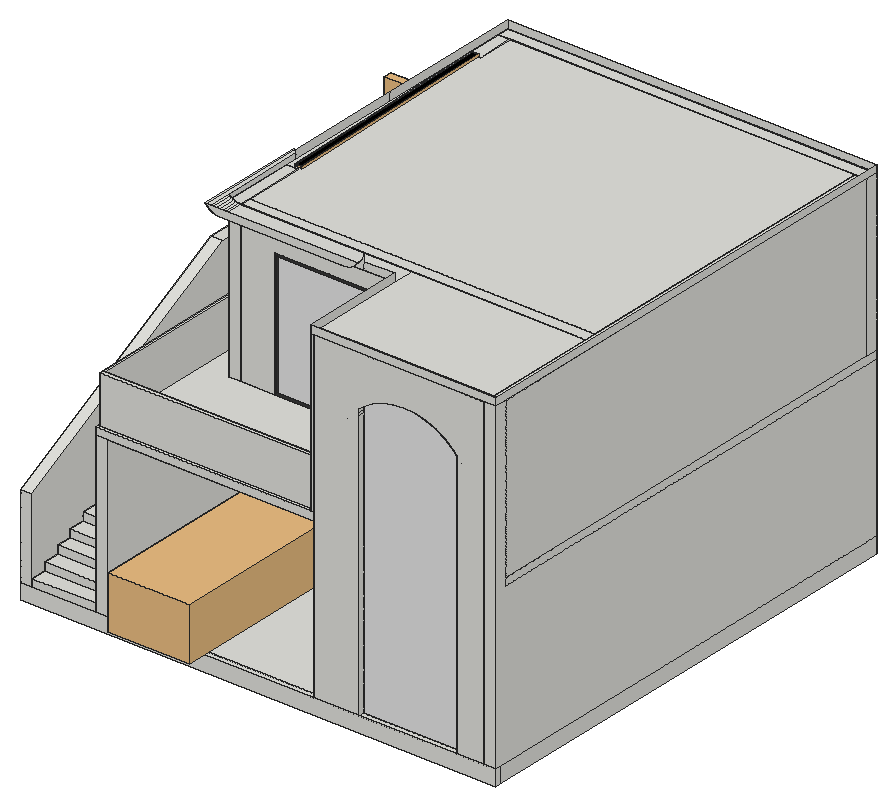
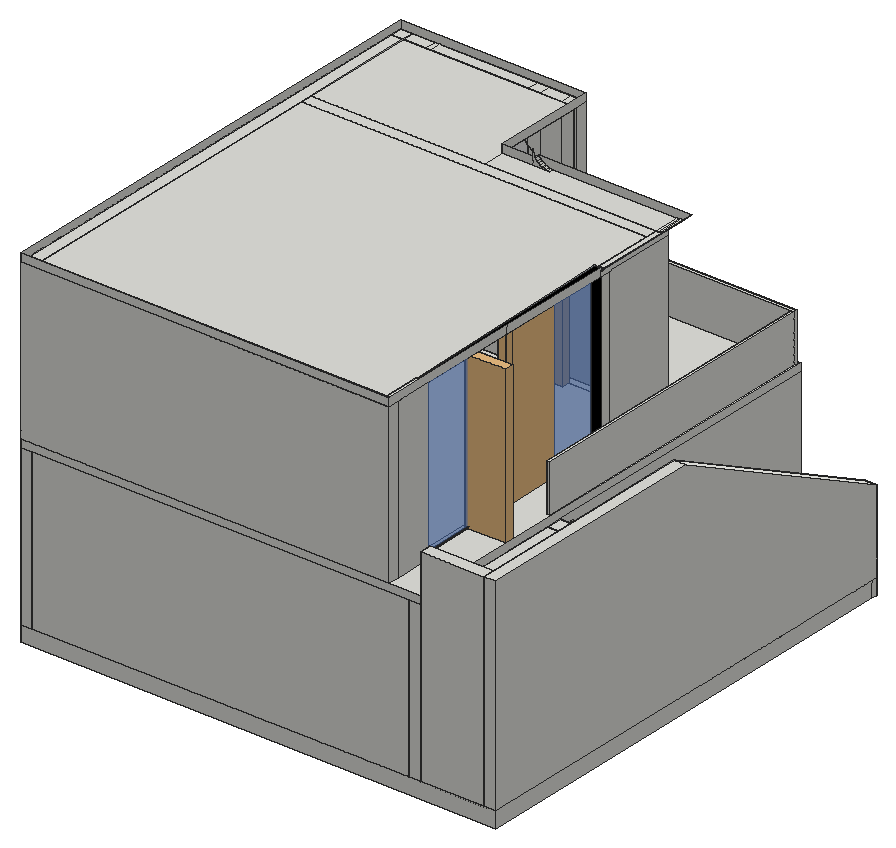
# SketchUp Ruby script. Lengths in inches.
U = 1.inch
M = Sketchup.active_model
def pt(a) = Geom::Point3d.new(a.map { |v| v * U })
def face(e, loops, mat)
  f = e.add_face(loops[0].map { |a| pt(a) })
  loops[1..].each { |l| e.add_face(l.map { |a| pt(a) }).erase! }
  f.material = f.back_material = mat if mat
  f
end
# faces: each face lists its corners as indices into pts; further lists are holes
def faces(e, pts, list, mat = nil) = list.each { |f| face(e, (f[0].is_a?(Array) ? f : [f]).map { |l| l.map { |i| pts[i] } }, mat) }
# xy, xz, yz: faces in a plane at the given z, y or x. An outline is a flat list of corners, or four numbers for a rectangle; further outlines are holes
def ring(l) = l.size == 4 ? [[l[0], l[1]], [l[2], l[1]], [l[2], l[3]], [l[0], l[3]]] : l.each_slice(2).to_a
def flat(e, list, mat, &to3) = list.each { |f| face(e, (f[0].is_a?(Array) ? f : [f]).map { |l| ring(l).map { |u, v| to3.(u, v) } }, mat) }
def xy(e, z, list, mat = nil) = flat(e, list, mat) { |x, y| [x, y, z] }
def xz(e, y, list, mat = nil) = flat(e, list, mat) { |x, z| [x, y, z] }
def yz(e, x, list, mat = nil) = flat(e, list, mat) { |y, z| [x, y, z] }
def lines(e, pts, list) = list.each { |a, b| e.add_line(pt(pts[a]), pt(pts[b])) }
# prism: a flat outline (further loops are holes) pulled along v
def prism(e, loops, v, mat = nil)
  f = face(e, loops, mat); d = Geom::Vector3d.new(v.map { |x| x * U })
  f.pushpull(f.normal.samedirection?(d) ? d.length : -d.length)
end
def box(e, o, s, mat = nil) = prism(e, [[o, [o[0] + s[0], o[1], o[2]], [o[0] + s[0], o[1] + s[1], o[2]], [o[0], o[1] + s[1], o[2]]]], [0, 0, s[2]], mat)
def at(x, y, z, deg = 0) = Geom::Transformation.translation(pt([x, y, z])) * Geom::Transformation.rotation(ORIGIN, Z_AXIS, deg.degrees)
def axes(o, x, y, z) = Geom::Transformation.new([*x, 0, *y, 0, *z, 0, *pt(o).to_a, 1])
def part(name) = M.definitions.add(name)
# library, detail: a bought-in or finely detailed component or shape, given as its bounding box
def library(name, o, s) = part(name).tap { |d| box(d.entities, o, s) }
def detail(e, o, s) = box(e.add_group.entities, o, s)
def put(e, d, t, mat = nil) = e.add_instance(d, t).tap { |i| i.material = mat if mat }
def group(e, t, mat = nil) = e.add_group.tap { |g| g.transformation = t; g.material = mat if mat }.entities
root = M.entities
M.materials.add("Color_006").color = [86, 86, 86]
M.materials.add("Metal_Aluminum_Anodized").color = [202, 209, 219]
M.materials.add("Translucent_Glass_Blue1").color = [0, 0, 0]
M.materials["Translucent_Glass_Blue1"].alpha = 0.15
M.materials.add("[Color M05]").color = [114, 114, 114]
M.materials.add("[Color M07]").color = [58, 58, 58]
M.materials.add("[Color M08]").color = [30, 30, 30]
M.materials.add("[Metal_Corrogated_Shiny]5").color = [0, 0, 0]
M.materials.add("[Mirror 01]").color = [185, 185, 185]
M.materials.add("[Mirror 02]").color = [229, 229, 229]
M.materials.add("[Translucent_Glass_Blue]").color = [100, 149, 237]
M.materials["[Translucent_Glass_Blue]"].alpha = 0.4
M.materials.add("[Wood Floor]").color = [155, 105, 61]
c1 = library("Curtains 003",[-24.98,-2.79,0.01],[49.96,5.58,117.31])
c2 = library("2016+Honda+Civic+LX+Sedan",[0.01,0.03,0.02],[16.17,34.46,10.62])
c3 = part("Flat washer")
detail(c3.entities,[0,0,0],[2.37,2.37,0.11])
c4 = part("Square cover plate")
detail(c4.entities,[0.66,9.07,0],[4.59,4.59,0.09])
c5 = part("Component\#60")
xy(c5.entities,0,[[1,0,4,4]],"[Metal_Corrogated_Shiny]5")
xy(c5.entities,0.95,[[1.17,0.17,3.83,3.83]],"[Metal_Corrogated_Shiny]5")
xy(c5.entities,3,[[[1,0,4,4],[1.17,0.17,3.83,3.83]]],"[Metal_Corrogated_Shiny]5")
xz(c5.entities,0,[[1,0,4,3]],"[Metal_Corrogated_Shiny]5")
xz(c5.entities,0.17,[[1.17,0.95,3.83,3]],"[Metal_Corrogated_Shiny]5")
xz(c5.entities,3.83,[[1.17,0.95,3.83,3]],"[Metal_Corrogated_Shiny]5")
xz(c5.entities,4,[[1,0,4,3]],"[Metal_Corrogated_Shiny]5")
yz(c5.entities,1,[[0,0,4,3]],"[Metal_Corrogated_Shiny]5")
yz(c5.entities,1.17,[[0.17,0.95,3.83,3]],"[Metal_Corrogated_Shiny]5")
yz(c5.entities,3.83,[[0.17,0.95,3.83,3]],"[Metal_Corrogated_Shiny]5")
yz(c5.entities,4,[[0,0,4,3]],"[Metal_Corrogated_Shiny]5")
c6 = part("Component\#28")
prism(c6.entities,[[[0.08,0.08,0],[0.04,0.13,0],[0.01,0.2,0],[0,0.27,0],[0.01,0.33,0],[0.04,0.4,0],[0.08,0.45,0],[0.13,0.5,0],[0.2,0.52,0],[0.27,0.53,0],[0.33,0.52,0],[0.4,0.5,0],[0.45,0.45,0],[0.5,0.4,0],[0.52,0.33,0],[0.53,0.27,0],[0.52,0.2,0],[0.5,0.13,0],[0.45,0.08,0],[0.4,0.04,0],[0.33,0.01,0],[0.27,0,0],[0.2,0.01,0],[0.13,0.04,0]]],[0,0,0.125])
c7 = part("Frame cover strip")
xz(c7.entities,0,[[0.0625,0,5.71,156]],"[Metal_Corrogated_Shiny]5")
xz(c7.entities,0.0625,[[0,0,0.0625,156],[5.71,0,5.78,156]])
xz(c7.entities,0.125,[[0,0,0.0625,156],[5.71,0,5.78,156]])
xz(c7.entities,0.1875,[[0,0,0.0625,156],[5.71,0,5.78,156]])
yz(c7.entities,0,[[0.0625,0,0.125,156]])
yz(c7.entities,0.0625,[[0,0,0.0625,156],[0.125,0,0.1875,156]])
yz(c7.entities,5.71,[[0,0,0.0625,156],[0.125,0,0.1875,156]])
yz(c7.entities,5.78,[[0.0625,0,0.125,156]])
c8 = part("Door frame channel")
detail(c8.entities,[0,0,0],[6.25,2.05,156])
c9 = part("Door frame channel \#1")
prism(c9.entities,[[[6.09,2,0],[6.09,1.625,0],[6.15,1.625,0],[6.15,0.125,0],[6.09,0.125,0],[6.09,0,0],[0.0625,0,0],[0.0625,0.125,0],[0,0.125,0],[0,1.625,0],[0.0625,1.625,0],[0.0625,2,0],[0.25,2,0],[5.9,2,0]],[[5.96,0.125,0],[5.96,1.875,0],[0.1875,1.875,0],[0.1875,0.125,0]]],[0,0,156],"[Metal_Corrogated_Shiny]5")
c10 = part("Component\#50")
box(c10.entities,[0,0,-3.25],[1.625,0.75,16.75])
c11 = part("Component\#53")
box(c11.entities,[0,0,0],[1.625,1,13.5],"[Metal_Corrogated_Shiny]5")
c12 = part("Component\#49")
xy(c12.entities,0,[[0.75,0,1.38,0.5]])
xy(c12.entities,16.75,[[0.75,0,1.38,0.5]])
xz(c12.entities,0,[[0.75,0,1.38,0,1.39,0.01,1.4,0,1.41,0.01,1.42,0,1.43,0.01,1.44,0,1.45,0.01,1.46,0,1.47,0.01,1.48,0,1.49,0.01,1.5,0,1.5,16.75,1.49,16.74,1.39,16.74,1.38,16.75,0.75,16.75],[1.39,16.74,1.41,16.74,1.4,16.75],[1.41,16.74,1.43,16.74,1.42,16.75],[1.43,16.74,1.45,16.74,1.44,16.75],[1.45,16.74,1.47,16.74,1.46,16.75],
  [1.47,16.74,1.49,16.74,1.48,16.75]])
xz(c12.entities,0.5,[[0.75,0,0.75,16.75,1.38,16.75,1.39,16.74,1.49,16.74,1.5,16.75,1.5,0,1.49,0.01,1.48,0,1.47,0.01,1.46,0,1.45,0.01,1.44,0,1.43,0.01,1.42,0,1.41,0.01,1.4,0,1.39,0.01,1.38,0],[1.39,16.74,1.4,16.75,1.41,16.74],[1.41,16.74,1.42,16.75,1.43,16.74],[1.43,16.74,1.44,16.75,1.45,16.74],[1.45,16.74,1.46,16.75,1.47,16.74],
  [1.47,16.74,1.48,16.75,1.49,16.74]])
yz(c12.entities,0.75,[[0,0,0.5,16.75]])
yz(c12.entities,1.5,[[0,0,0.5,16.75]])
p = [[1.38,0.5,0],[1.39,0.5,0.01],[1.39,0,0.01],[1.38,0,0],[1.4,0.5,0],[1.4,0,0],
  [1.41,0.5,0.01],[1.41,0,0.01],[1.42,0.5,0],[1.42,0,0],[1.43,0.5,0.01],[1.43,0,0.01],
  [1.44,0.5,0],[1.44,0,0],[1.45,0.5,0.01],[1.45,0,0.01],[1.46,0.5,0],[1.46,0,0],
  [1.47,0.5,0.01],[1.47,0,0.01],[1.48,0.5,0],[1.48,0,0],[1.49,0.5,0.01],[1.49,0,0.01],
  [1.5,0.5,0],[1.5,0,0],[1.46,0.5,16.75],[1.45,0.5,16.74],[1.45,0,16.74],[1.46,0,16.75],
  [1.44,0.5,16.75],[1.44,0,16.75],[1.43,0.5,16.74],[1.43,0,16.74],[1.42,0.5,16.75],[1.42,0,16.75],
  [1.41,0.5,16.74],[1.41,0,16.74],[1.4,0.5,16.75],[1.4,0,16.75],[1.39,0.5,16.74],[1.39,0,16.74],
  [1.38,0.5,16.75],[1.38,0,16.75],[1.5,0.5,16.75],[1.49,0.5,16.74],[1.49,0,16.74],[1.5,0,16.75],
  [1.48,0.5,16.75],[1.48,0,16.75],[1.47,0.5,16.74],[1.47,0,16.74]]
faces(c12.entities,p,[[0,1,2,3],[1,4,5,2],[4,6,7,5],[6,8,9,7],[8,10,11,9],[10,12,13,11],[12,14,15,13],[14,16,17,15],
  [16,18,19,17],[18,20,21,19],[20,22,23,21],[22,24,25,23],[26,27,28,29],[27,30,31,28],[30,32,33,31],[32,34,35,33],
  [34,36,37,35],[36,38,39,37],[38,40,41,39],[40,42,43,41],[44,45,46,47],[45,48,49,46],[48,50,51,49],[50,26,29,51]])
c13 = library("Glass door assembly",[0,0.34,0.3125],[36,6.07,85.9375])
c14 = part("Glazing strip")
prism(c14.entities,[[[0,0,0],[0,0.375,0],[0.61,0.375,0],[0.61,0,0],[0.55,0,0],[0.55,0.24,0],[0.49,0.31,0],[0.12,0.31,0],[0.05,0.24,0],[0.05,0,0]]],[0,0,36])
c15 = part("Glazing rail")
prism(c15.entities,[[[0,0,0],[0,0.75,0],[0.75,0.75,0],[0.75,0,0],[0.68,0,0],[0.68,0.375,0],[0.07,0.375,0],[0.07,0,0]]],[0,0,36])
c16 = part("Glass pane")
prism(c16.entities,[[[0.0625,83.11,0],[0.4375,83.11,0],[0.5,83.05,0],[0.5,0.0625,0],[0.4375,0,0],[0.0625,0,0],[0,0.0625,0],[0,83.05,0]]],[0,0,36],"[Translucent_Glass_Blue]")
c17 = part("Glazing rail \#1")
prism(c17.entities,[[[0,0,0],[0,1,0],[0.75,1,0],[0.75,0,0],[0.68,0,0],[0.68,0.375,0],[0.07,0.375,0],[0.07,0,0]]],[0,0,36],"[Metal_Corrogated_Shiny]5")
c18 = part("Fixed glass panel \#1")
put(c18.entities,c14,axes([0,2.57,0.75],[0,1,0],[0,0,-1],[1,0,0]),"Color_006")
put(c18.entities,c15,axes([0,2.5,0.75],[0,1,0],[0,0,-1],[1,0,0]),"Metal_Aluminum_Anodized")
put(c18.entities,c16,axes([0,2.625,0.44],[0,1,0],[0,0,1],[1,0,0]),"Translucent_Glass_Blue1")
put(c18.entities,c14,axes([0,2.57,83.25],[0,1,0],[0,0,1],[1,0,0]),"Color_006")
put(c18.entities,c17,axes([0,2.5,83.25],[0,1,0],[0,0,1],[1,0,0]),"Metal_Aluminum_Anodized")
c19 = part("Component\#21")
box(c19.entities,[0,0,0.5],[1.5,0.5,0.1875],"Metal_Aluminum_Anodized")
c20 = part("Fixed glass panel")
put(c20.entities,c18,at(0,-2.5,1))
put(c20.entities,c19,at(1.24,0.125,0.3125))
put(c20.entities,c19,at(33.41,0.125,0.3125))
c21 = part("Glass Doors")
p = [[-9.64,246.33,0],[-9.66,246.34,0],[-9.64,246.35,0],[-9.66,246.36,0],[-9.64,246.375,0],[-9.66,246.38,0],
  [-9.64,246.39,0],[-9.66,246.4,0],[-9.64,246.41,0],[-9.66,246.42,0],[-9.64,246.43,0],[-9.66,246.44,0],
  [-9.64,246.45,0]]
lines(c21.entities,p,[[0,1],[1,2],[2,3],[3,4],[4,5],[5,6],[6,7],[7,8],[8,9],[9,10],[10,11],[11,12]])
put(c21.entities,c3,axes([131.42,22.72,-1.61],[0,-1,0],[-1,0,0],[0,0,1]))
put(c21.entities,c4,axes([141.61,24.49,0],[0,-1,0],[-1,0,0],[0,0,1]),"Metal_Aluminum_Anodized")
put(c21.entities,c3,axes([62.98,22.72,-1.61],[0,-1,0],[-1,0,0],[0,0,1]))
put(c21.entities,c4,axes([73.16,24.49,0],[0,-1,0],[-1,0,0],[0,0,1]),"Metal_Aluminum_Anodized")
put(c21.entities,c5,at(59.79,23.6,-3,-90),"Metal_Aluminum_Anodized")
put(c21.entities,c5,at(128.05,23.6,-3,-90),"Metal_Aluminum_Anodized")
put(c21.entities,c3,axes([131.24,22.29,-1.61],[0,-1,0],[-1,0,0],[0,0,1]))
put(c21.entities,c6,at(57.64,21.27,84.4375))
put(c21.entities,c7,axes([18.08,18.65,86.62],[0,1,0],[0,0,1],[1,0,0]),"Metal_Aluminum_Anodized")
put(c21.entities,c8,axes([18.08,18.41,84.5625],[0,1,0],[0,0,1],[1,0,0]),"Metal_Aluminum_Anodized")
put(c21.entities,c9,axes([18.08,18.46,84.62],[0,1,0],[0,0,1],[1,0,0]),"Metal_Aluminum_Anodized")
put(c21.entities,c10,axes([90.95,18.76,83.8125],[0,1,0],[0,0,1],[1,0,0]),"Color_006")
put(c21.entities,c6,at(133.86,21.27,84.4375))
put(c21.entities,c6,at(61.68,21.27,84.4375))
put(c21.entities,c11,axes([118.42,21.99,83.4375],[0,1,0],[0,0,1],[1,0,0]),"Color_006")
put(c21.entities,c11,axes([60.11,21.99,83.4375],[0,1,0],[0,0,1],[1,0,0]),"Color_006")
put(c21.entities,c6,at(129.83,21.27,84.4375))
put(c21.entities,c12,axes([87.7,19.63,83.9375],[0,1,0],[0,0,1],[1,0,0]))
put(c21.entities,c13,at(58.58,23.52,-1.8125,-90))
put(c21.entities,c20,at(23.83,21.16,-0.8125))
put(c21.entities,c20,at(132.2,21.16,-0.8125))
put(c21.entities,c13,axes([132.08,18.32,-1.8125],[-1,0,0],[0,1,0],[0,0,1]))
c22 = part("Glass Door")
p = [[29.51,29.22,3.1875],[24.38,26.97,3.1875],[24.38,26.97,87.4375],[29.51,29.22,87.4375],[159.55,32.17,87.4375],[164.89,30.16,87.4375],
  [164.89,30.16,3.1875],[159.55,32.17,3.1875]]
faces(c22.entities,p,[[0,1,2,3],[4,5,6,7]],"[Metal_Corrogated_Shiny]5")
put(c22.entities,c21,axes([8.46,10.78,3],[0.9007,0.02044,0],[-0.01925,0.84838,0],[0,0,1]),"[Metal_Corrogated_Shiny]5")
xy(root,-12,[[0,0,360,4.03],[0,4.03,360,360]])
xy(root,0,[[0,0,9,4.03],[9,0,57,4.03],[57,0,66,4.03],[66,0,222,4.03],[222,0,256.5,4.03],
  [256.5,0,330.23,4.03],[330.23,0,351,4.03],[351,0,360,4.03],[0,4.03,9,360],[9,4.03,57,240],
  [57,4.03,66,360],[66,4.03,222,129],[222,4.03,256.5,4.03,256.5,4.5,330.23,4.5,330.23,9,231,9,231,138,160.73,138,160.73,129,222,129],[222,4.03,256.5,9],[256.5,4.03,330.23,4.5],
  [330.23,4.03,351,9],[351,4.03,360,360],[256.5,4.5,330.23,5.75],[256.5,5.75,330.23,9],[231,9,351,9,351,351,66,351,66,138,231,138],
  [222,9,231,138],[66,129,160.73,138],[160.73,129,222,133.5],[160.73,137.0625,222,138],[9,240,57,350.8],
  [9,350.8,57,360],[66,351,351,360]])
xy(root,0,[[160.73,133.5,222,137.0625]],"[Color M07]")
xy(root,3.46,[[164.19,133.5,188.9,135.1875],[191.36,133.5,218.54,135.1875]],"[Color M07]")
xy(root,6,[[9,0,57,12]])
xy(root,12,[[9,12,57,24]])
xy(root,18,[[9,24,57,36]])
xy(root,24,[[9,36,57,48]])
xy(root,30,[[9,48,57,60]])
xy(root,36,[[9,60,57,72]])
xy(root,42,[[9,72,57,84]])
xy(root,48,[[9,84,57,96]])
xy(root,54,[[9,96,57,108]])
xy(root,60,[[9,108,57,120]])
xy(root,66,[[9,120,57,132]])
xy(root,72,[[9,132,57,144]])
xy(root,78,[[9,144,57,156]])
xy(root,84,[[9,156,57,168]])
xy(root,90,[[9,168,57,180]])
xy(root,96,[[9,180,57,192]])
xy(root,102,[[9,192,57,204]])
xy(root,108,[[9,204,57,216]])
xy(root,114,[[9,216,57,228]])
xy(root,116.54,[[164.19,133.5,188.9,135.1875],[191.36,133.5,218.54,135.1875]],"[Color M07]")
xy(root,120,[[57,0,66,360],[66,0,66,129,160.73,129,160.73,133.5,222,133.5,222,0],[231,9,231,138,222,138,222,137.0625,160.73,137.0625,160.73,138,66,138,66,351,351,351,351,9],[222,9,231,138],[351,9,360,360],
  [66,129,160.73,138],[160.73,133.5,222,137.0625],[9,228,57,240],[9,240,57,350.8],[66,351,351,360]])
xy(root,120,[[160.73,133.5,222,137.0625]],"[Color M07]")
xy(root,126,[[57,0,219.5625,0,219.5625,2.33,58.46,2.33,58.46,235.98,60.8125,235.98,60.8125,5.1875,219.5625,5.1875,219.5625,9,351,9,351,96,81,96,81,150.52,90,150.52,90,322.98,81,322.98,81,360,57,360],[219.5625,0,222,2.33],[58.46,2.33,219.5625,5.1875],[219.5625,2.33,222,5.1875],[58.46,5.1875,60.8125,235.98],
  [219.5625,5.1875,222,9],[351,9,360,351],[81,96,90,150.52],[90,96,115.87,105],[193.03,96,272.01,105],
  [332.47,96,351,105],[272.01,97.625,332.47,105],[115.87,99.1875,193.03,105],[90,105,351,351],[81,322.98,90,351],
  [81,351,360,360]])
xy(root,126,[[115.87,96,193.03,99.1875]],"[Color M07]")
xy(root,126,[[272.01,96,332.47,97.625]],"[Color M08]")
xy(root,127.5625,[[117.43,96,191.46,96.75]],"[Color M07]")
xy(root,129.19,[[275.2,96,329.27,96.0625]])
xy(root,156,[[0,180,9,360],[9,350.8,57,360]])
xy(root,162,[[58.46,2.33,219.5625,5.1875],[58.46,5.1875,60.8125,235.98]])
xy(root,218.81,[[275.2,96,329.27,96.0625]])
xy(root,220.4375,[[117.43,96,191.46,96.75]],"[Color M07]")
xy(root,222,[[272.01,97.625,332.47,105],[115.87,99.1875,193.03,105]])
xy(root,222,[[115.87,96,193.03,99.1875]],"[Color M07]")
xy(root,222,[[272.01,96,332.47,97.625]],"[Color M08]")
xy(root,246,[[219.5625,0,222,9],[222,0,231,9],[231,0,247.4375,9],[247.4375,0,256.5,9],[256.5,0,330.23,9],
  [330.23,0,333.6,9],[333.6,0,351,9],[351,0,360,9],[219.5625,9,351,96],[351,9,360,351],
  [90,76.3125,90,96,219.5625,96,219.5625,79.5,183.54,79.5,183.54,76.3125],[81,96,90,150.52],[90,96,351,105],[90,105,90,150.52,81,150.52,81,322.98,90,322.98,90,351,351,351,351,105],[81,322.98,90,351],
  [81,351,360,360]])
xz(root,0,[[0,-12,360,0],[0,0,9,63.0625],[9,0,57,6],[57,0,66,120],[222,0,256.5,0,256.5,207.79,259.09,210.07,266.21,214.56,273.96,217.85,282.13,219.86,290.52,220.53,298.91,219.86,307.08,217.85,314.83,214.56,321.95,210.07,328.26,204.51,330.23,202.11,330.23,0,351,0,351,246,222,246],
  [351,0,360,246],[57,120,222,126],[219.5625,126,222,246],[219.5625,246,360,252]])
xz(root,2.33,[[58.46,126,219.5625,162]])
xz(root,4.03,[[0,-12,360,0]])
xz(root,4.5,[[256.5,0,330.23,0,330.23,202.11,328.26,204.51,321.95,210.07,314.83,214.56,307.08,217.85,298.91,219.86,290.52,220.53,282.13,219.86,273.96,217.85,266.21,214.56,259.09,210.07,256.5,207.79]],"[Mirror 02]")
xz(root,5.1875,[[58.46,126,60.8125,162],[60.8125,126,219.5625,162]])
xz(root,5.75,[[256.5,0,256.5,207.79,259.09,210.07,266.21,214.56,273.96,217.85,282.13,219.86,290.52,220.53,298.91,219.86,307.08,217.85,314.83,214.56,321.95,210.07,328.26,204.51,330.23,202.11,330.23,0]],"[Mirror 02]")
xz(root,9,[[222,0,231,120],[231,0,256.5,120],[256.5,0,330.23,120],[330.23,0,351,120],[222,120,231,126],
  [231,120,256.5,126],[256.5,120,330.23,126],[330.23,120,351,126],[351,120,360,126],[219.5625,126,222,246],
  [222,126,231,246],[231,126,256.5,126,256.5,207.79,252.78,204.51,247.4375,198,247.4375,246,231,246],[330.23,126,330.23,202.11,333.6,198,333.6,246,351,246,351,126],[351,126,360,246],[247.4375,198,247.4375,246,256.5,246,256.5,207.79,252.78,204.51],
  [333.6,198,330.23,202.11,330.23,246,333.6,246],[330.23,202.11,328.26,204.51,321.95,210.07,314.83,214.56,307.08,217.85,298.91,219.86,290.52,220.53,282.13,219.86,273.96,217.85,266.21,214.56,259.09,210.07,256.5,207.79,256.5,246,330.23,246]])
xz(root,12,[[9,6,57,12]])
xz(root,24,[[9,12,57,18]])
xz(root,36,[[9,18,57,24]])
xz(root,48,[[9,24,57,30]])
xz(root,60,[[9,30,57,36]])
xz(root,72,[[9,36,57,42]])
xz(root,76.3125,[[90,246,183.54,246,185.08,246.09,186.6,246.36,188.07,246.8,189.49,247.41,190.82,248.18,192.06,249.1,193.17,250.16,194.16,251.35,194.59,252,78.98,252,79.54,251.16,80.68,249.86,81.97,248.73,83.41,247.77,84.95,247,86.59,246.45,88.28,246.11]])
xz(root,79.5,[[183.54,246,196.57,246,196.57,256.96,196.22,255.46,195.69,254.01,195.01,252.63,194.59,252,194.16,251.35,193.17,250.16,192.06,249.1,190.82,248.18,189.49,247.41,188.07,246.8,186.6,246.36,185.08,246.09],[196.57,246,219.5625,252]])
xz(root,84,[[9,42,57,48]])
xz(root,96,[[9,48,57,54],[81,126,90,246],[90,126,115.87,126,115.87,222,193.03,222,193.03,126,272.01,126,272.01,222,332.47,222,332.47,126,351,126,351,246,90,246],[81,246,90,246,88.28,246.11,86.59,246.45,84.95,247,83.41,247.77,81.97,248.73,81,249.58]])
xz(root,96,[[[115.87,126,193.03,222],[117.43,127.5625,191.46,220.4375]]],"[Color M07]")
xz(root,96,[[[272.01,126,332.47,222],[275.2,129.19,329.27,218.81]]],"[Color M08]")
xz(root,96.0625,[[275.2,129.19,329.27,218.81]],"[Wood Floor]")
xz(root,96.75,[[117.43,127.5625,191.46,220.4375]],"[Mirror 02]")
xz(root,97.625,[[272.01,126,332.47,222]])
xz(root,99.1875,[[115.87,126,193.03,222]],"[Mirror 02]")
xz(root,105,[[90,126,90,246,351,246,351,126,332.47,126,332.47,222,272.01,222,272.01,126,193.03,126,193.03,222,115.87,222,115.87,126]])
xz(root,108,[[9,54,57,60]])
xz(root,120,[[9,60,57,66]])
xz(root,129,[[66,0,160.73,120]])
xz(root,132,[[9,66,57,72]])
xz(root,133.5,[[[160.73,0,222,120],[164.19,3.46,218.54,116.54]],[188.9,3.46,191.36,116.54]],"[Color M07]")
xz(root,135.1875,[[164.19,3.46,188.9,116.54],[191.36,3.46,218.54,116.54]],"[Mirror 01]")
xz(root,137.0625,[[160.73,0,222,120]],"[Mirror 01]")
xz(root,138,[[66,0,160.73,120],[222,0,231,120]])
xz(root,144,[[9,72,57,78]])
xz(root,150.52,[[81,126,90,246]])
xz(root,156,[[9,78,57,84]])
xz(root,159.75,[[81,249.58,80.68,249.86,79.54,251.16,78.98,252,81,252]])
xz(root,168,[[9,84,57,90]])
xz(root,180,[[9,90,57,96]])
xz(root,192,[[9,96,57,102]])
xz(root,204,[[9,102,57,108]])
xz(root,216,[[9,108,57,114]])
xz(root,228,[[9,114,57,120]])
xz(root,235.98,[[58.46,126,60.8125,162]])
xz(root,240,[[9,0,57,120]])
xz(root,322.98,[[81,126,90,246]])
xz(root,350.8,[[9,0,57,120],[9,120,57,156]])
xz(root,351,[[66,0,351,120],[81,126,90,246],[90,126,351,246],[351,126,360,246]])
xz(root,360,[[0,-12,360,0],[0,0,9,156],[9,0,57,156],[57,0,66,120],[66,0,351,120],
  [351,0,360,120],[57,120,360,126],[81,126,360,246],[81,246,360,252]])
yz(root,0,[[0,-12,4.03,0],[4.03,-12,360,0],[0,0,0,63.0625,180,156,360,156,360,0]])
yz(root,9,[[0,0,240,0,240,120,228,120,228,114,216,114,216,108,204,108,204,102,192,102,192,96,180,96,180,90,168,90,168,84,156,84,156,78,144,78,144,72,132,72,132,66,120,66,120,60,108,60,108,54,96,54,96,48,84,48,84,42,72,42,72,36,60,36,60,30,48,30,48,24,36,24,36,18,24,18,24,12,12,12,12,6,0,6],[240,0,350.8,120],[350.8,0,360,156],[0,6,12,6,12,12,24,12,24,18,36,18,36,24,48,24,48,30,60,30,60,36,72,36,72,42,84,42,84,48,96,48,96,54,108,54,108,60,120,60,120,66,132,66,132,72,144,72,144,78,156,78,156,84,168,84,168,90,180,90,180,96,192,96,192,102,204,102,204,108,216,108,216,114,228,114,228,156,180,156,0,63.0625],[228,120,240,156],
  [240,120,350.8,156]])
yz(root,57,[[0,0,240,0,240,120,228,120,228,114,216,114,216,108,204,108,204,102,192,102,192,96,180,96,180,90,168,90,168,84,156,84,156,78,144,78,144,72,132,72,132,66,120,66,120,60,108,60,108,54,96,54,96,48,84,48,84,42,72,42,72,36,60,36,60,30,48,30,48,24,36,24,36,18,24,18,24,12,12,12,12,6,0,6],[240,0,350.8,120],[350.8,0,360,120],[0,6,0,120,228,120,228,114,216,114,216,108,204,108,204,102,192,102,192,96,180,96,180,90,168,90,168,84,156,84,156,78,144,78,144,72,132,72,132,66,120,66,120,60,108,60,108,54,96,54,96,48,84,48,84,42,72,42,72,36,60,36,60,30,48,30,48,24,36,24,36,18,24,18,24,12,12,12,12,6],[0,120,350.8,126],
  [350.8,120,360,126],[350.8,126,360,156]])
yz(root,58.46,[[2.33,126,5.1875,162],[5.1875,126,235.98,162]])
yz(root,60.8125,[[5.1875,126,235.98,162]])
yz(root,66,[[0,0,129,120],[129,0,138,120],[138,0,351,120],[351,0,360,120]])
yz(root,81,[[96,126,150.52,246],[322.98,126,351,246],[351,126,360,246],[96,246,159.75,249.58],[159.75,246,248.24,252],
  [248.24,246,360,252]])
yz(root,90,[[96,126,105,246],[105,126,150.52,246],[322.98,126,351,246]])
yz(root,115.87,[[99.1875,126,105,222]])
yz(root,115.87,[[96,126,99.1875,222]],"[Color M07]")
yz(root,117.43,[[96,127.5625,96.75,220.4375]],"[Color M07]")
yz(root,160.73,[[129,0,133.5,120],[137.0625,0,138,120]])
yz(root,160.73,[[133.5,0,137.0625,120]],"[Color M07]")
yz(root,164.19,[[133.5,3.46,135.1875,116.54]],"[Color M07]")
yz(root,188.9,[[133.5,3.46,135.1875,116.54]],"[Color M07]")
yz(root,191.36,[[133.5,3.46,135.1875,116.54]],"[Color M07]")
yz(root,191.46,[[96,127.5625,96.75,220.4375]],"[Color M07]")
yz(root,193.03,[[99.1875,126,105,222]])
yz(root,193.03,[[96,126,99.1875,222]],"[Color M07]")
yz(root,218.54,[[133.5,3.46,135.1875,116.54]],"[Color M07]")
yz(root,219.5625,[[0,126,0,246,9,246,9,126,5.1875,126,5.1875,162,2.33,162,2.33,126],[2.33,126,5.1875,162],[0,246,79.5,252]])
yz(root,222,[[0,0,9,120],[9,0,129,120],[129,0,133.5,120],[137.0625,0,138,120],[0,120,9,126],
  [0,126,9,246]])
yz(root,222,[[133.5,0,137.0625,120]],"[Color M07]")
yz(root,231,[[9,0,138,120]])
yz(root,256.5,[[0,0,4.5,203.13],[4.5,0,5.75,203.13],[5.75,0,9,203.13],[0,203.13,4.5,205.46],[4.5,203.13,5.75,205.46],
  [5.75,203.13,9,205.46],[0,205.46,4.5,207.79],[4.5,205.46,5.75,207.79],[5.75,205.46,9,207.79]])
yz(root,272.01,[[97.625,126,105,222]])
yz(root,272.01,[[96,126,97.625,222]],"[Color M08]")
yz(root,275.2,[[96,129.19,96.0625,218.81]])
yz(root,329.27,[[96,129.19,96.0625,218.81]])
yz(root,330.23,[[0,0,4.5,198.18],[4.5,0,5.75,202.11],[0,198.18,4.5,202.11]])
yz(root,332.47,[[97.625,126,105,222]])
yz(root,332.47,[[96,126,97.625,222]],"[Color M08]")
yz(root,351,[[0,0,9,246],[9,0,351,120],[351,0,360,120],[9,126,96,246],[96,126,105,246],
  [105,126,351,246]])
yz(root,360,[[0,-12,4.03,0],[4.03,-12,360,0],[0,0,360,0,360,120,9,120,9,246,0,246],[9,120,360,126],[9,126,351,246],
  [351,126,360,246],[0,246,360,252]])
p = [[0,180,156],[0,0,63.0625],[9,0,63.0625],[9,180,156],[330.23,4.5,202.11],[330.23,0,202.11],
  [328.26,0,204.51],[328.26,4.5,204.51],[328.26,5.75,204.51],[330.23,5.75,202.11],[321.95,0,210.07],[321.95,4.5,210.07],
  [321.95,5.75,210.07],[328.26,9,204.51],[321.95,9,210.07],[256.5,0,207.79],[256.5,4.5,207.79],[259.09,4.5,210.07],
  [259.09,0,210.07],[259.09,5.75,210.07],[256.5,5.75,207.79],[259.09,9,210.07],[256.5,9,207.79],[266.21,4.5,214.56],
  [266.21,0,214.56],[314.83,0,214.56],[314.83,4.5,214.56],[266.21,5.75,214.56],[314.83,5.75,214.56],[266.21,9,214.56],
  [314.83,9,214.56],[273.96,4.5,217.85],[273.96,0,217.85],[307.08,0,217.85],[307.08,4.5,217.85],[273.96,5.75,217.85],
  [307.08,5.75,217.85],[273.96,9,217.85],[307.08,9,217.85],[282.13,4.5,219.86],[282.13,0,219.86],[298.91,0,219.86],
  [298.91,4.5,219.86],[282.13,5.75,219.86],[298.91,5.75,219.86],[282.13,9,219.86],[298.91,9,219.86],[290.52,4.5,220.53],
  [290.52,0,220.53],[290.52,5.75,220.53],[290.52,9,220.53],[90,76.3125,246],[88.28,76.3125,246.11],[88.28,96,246.11],
  [90,96,246],[185.08,76.3125,246.09],[183.54,76.3125,246],[183.54,79.5,246],[185.08,79.5,246.09],[86.59,76.3125,246.45],
  [86.59,96,246.45],[186.6,76.3125,246.36],[186.6,79.5,246.36],[84.95,76.3125,247],[84.95,96,247],[188.07,76.3125,246.8],
  [188.07,79.5,246.8],[189.49,76.3125,247.41],[189.49,79.5,247.41],[83.41,76.3125,247.77],[83.41,96,247.77],[190.82,76.3125,248.18],
  [190.82,79.5,248.18],[81.97,76.3125,248.73],[81.97,96,248.73],[192.06,76.3125,249.1],[192.06,79.5,249.1],[80.68,76.3125,249.86],
  [80.68,159.75,249.86],[81,159.75,249.58],[81,96,249.58],[193.17,76.3125,250.16],[193.17,79.5,250.16],[79.54,76.3125,251.16],
  [79.54,159.75,251.16],[194.16,76.3125,251.35],[194.16,79.5,251.35],[78.98,76.3125,252],[78.98,159.75,252],[194.59,76.3125,252],
  [194.59,79.5,252],[247.4375,0,198],[247.4375,9,198],[333.6,0,198],[333.6,9,198]]
faces(root,p,[[0,1,2,3],[4,5,6,7],[4,7,8,9],[10,11,7,6],[11,7,8,12],[13,8,12,14],[15,16,17,18],[16,17,19,20],
  [21,19,20,22],[18,17,23,24],[25,26,11,10],[17,23,27,19],[26,11,12,28],[29,27,19,21],[14,12,28,30],[24,23,31,32],
  [33,34,26,25],[23,31,35,27],[34,26,28,36],[37,35,27,29],[30,28,36,38],[32,31,39,40],[41,42,34,33],[31,39,43,35],
  [42,34,36,44],[45,43,35,37],[38,36,44,46],[40,39,47,48],[48,47,42,41],[39,47,49,43],[47,42,44,49],[50,49,43,45],
  [46,44,49,50],[51,52,53,54],[55,56,57,58],[52,59,60,53],[61,55,58,62],[59,63,64,60],[65,61,62,66],[67,65,66,68],
  [63,69,70,64],[71,67,68,72],[69,73,74,70],[75,71,72,76],[73,77,78,79,80,74],[81,75,76,82],[77,83,84,78],[85,81,82,86],
  [83,87,88,84],[89,85,86,90]])
lines(root,p,[[91,92],[93,94]])
put(root,c1,at(196.3125,138,0),"[Color M05]")
put(root,c1,at(308.99,9,0),"[Color M05]")
put(root,c2,axes([77.89,-14.53,-0.0625],[3.81,0,0],[0,3.81,0],[0,0,3.81]))
put(root,c22,axes([56.03,353.7,121.25],[0,-1.22,0],[1,0,0],[0,0,1.40304]))
put(root,c1,at(173.46,107.79,125.99),"[Color M05]")
put(root,c1,at(308.99,9,126),"[Color M05]")
